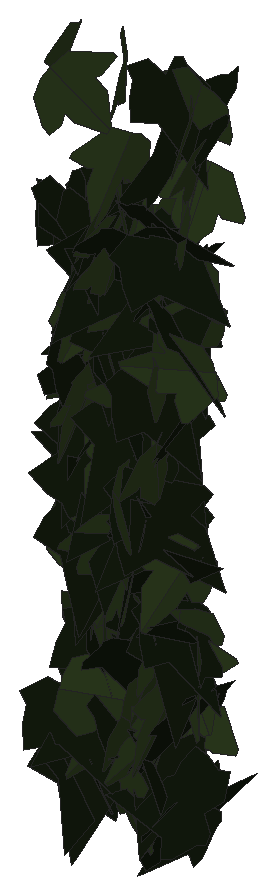
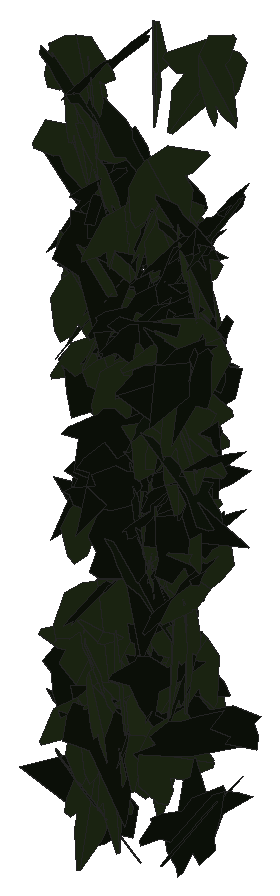
# SketchUp Ruby script. Lengths in inches.
U = 1.inch
M = Sketchup.active_model
def pt(a) = Geom::Point3d.new(a.map { |v| v * U })
def face(e, loops, mat)
  f = e.add_face(loops[0].map { |a| pt(a) })
  loops[1..].each { |l| e.add_face(l.map { |a| pt(a) }).erase! }
  f.material = f.back_material = mat if mat
  f
end
# faces: each face lists its corners as indices into pts; further lists are holes
def faces(e, pts, list, mat = nil) = list.each { |f| face(e, (f[0].is_a?(Array) ? f : [f]).map { |l| l.map { |i| pts[i] } }, mat) }
# xy, xz, yz: faces in a plane at the given z, y or x. An outline is a flat list of corners, or four numbers for a rectangle; further outlines are holes
def ring(l) = l.size == 4 ? [[l[0], l[1]], [l[2], l[1]], [l[2], l[3]], [l[0], l[3]]] : l.each_slice(2).to_a
def flat(e, list, mat, &to3) = list.each { |f| face(e, (f[0].is_a?(Array) ? f : [f]).map { |l| ring(l).map { |u, v| to3.(u, v) } }, mat) }
def xy(e, z, list, mat = nil) = flat(e, list, mat) { |x, y| [x, y, z] }
def xz(e, y, list, mat = nil) = flat(e, list, mat) { |x, z| [x, y, z] }
def yz(e, x, list, mat = nil) = flat(e, list, mat) { |y, z| [x, y, z] }
def lines(e, pts, list) = list.each { |a, b| e.add_line(pt(pts[a]), pt(pts[b])) }
# prism: a flat outline (further loops are holes) pulled along v
def prism(e, loops, v, mat = nil)
  f = face(e, loops, mat); d = Geom::Vector3d.new(v.map { |x| x * U })
  f.pushpull(f.normal.samedirection?(d) ? d.length : -d.length)
end
def box(e, o, s, mat = nil) = prism(e, [[o, [o[0] + s[0], o[1], o[2]], [o[0] + s[0], o[1] + s[1], o[2]], [o[0], o[1] + s[1], o[2]]]], [0, 0, s[2]], mat)
def at(x, y, z, deg = 0) = Geom::Transformation.translation(pt([x, y, z])) * Geom::Transformation.rotation(ORIGIN, Z_AXIS, deg.degrees)
def axes(o, x, y, z) = Geom::Transformation.new([*x, 0, *y, 0, *z, 0, *pt(o).to_a, 1])
def part(name) = M.definitions.add(name)
# library, detail: a bought-in or finely detailed component or shape, given as its bounding box
def library(name, o, s) = part(name).tap { |d| box(d.entities, o, s) }
def detail(e, o, s) = box(e.add_group.entities, o, s)
def put(e, d, t, mat = nil) = e.add_instance(d, t).tap { |i| i.material = mat if mat }
def group(e, t, mat = nil) = e.add_group.tap { |g| g.transformation = t; g.material = mat if mat }.entities
root = M.entities
M.materials.add("efeu1").color = [18, 25, 13]
M.materials.add("efeu2").color = [43, 57, 29]
c1 = part("ivyleaf_10")
p = [[0,0.5,-0.03],[-0.0625,2.02,-0.43],[-0.19,2.01,-0.46],[-0.54,1.05,-0.29],[-0.52,0.625,-0.18],[-0.83,0.76,-0.28],
  [-1.16,0.64,-0.33],[-1.15,0.33,-0.24],[-0.77,-0.39,0.02],[-0.3,-0.51,0.16],[0.04,-0.48,0.23],[-0.02,2.01,-0.4375],
  [-0.06,2.01,-0.43],[0.04,-0.49,0.23],[0.67,-0.49,0.14],[1.38,0.36,-0.2],[1.375,0.51,-0.24],[0.81,0.65,-0.19],
  [0.62,0.59,-0.15],[0.6,1.09,-0.28],[0.5,1.23,-0.31]]
faces(c1.entities,p,[[0,1,2,3,4,5,6,7,8,9,10],[11,12,0,13,14,15,16,17,18,19,20]],"efeu2")
c2 = part("ivyleaf_9")
p = [[1.54,2.16,1.25],[1.36,2.04,1.19],[-0.21,0.99,0.68],[-0.71,1.11,0.82],[-0.85,0.86,0.67],[-0.8,0.17,0.21],
  [-0.9,-0.01,0.1],[-0.67,-0.16,-0.02],[-0.08,-0.08,-0.05],[-0.03,-0.6,-0.4],[0.65,-0.88,-0.66],[0.83,-0.6,-0.49],
  [1.29,-0.42,-0.43],[1.8125,-0.07,-0.26],[1.21,0.44,0.15]]
faces(c2.entities,p,[[0,1,2,3,4,5,6,7,8,9,10,11,12,13,14]],"efeu1")
put(root,c1,axes([29.95,223.1,233.6],[0.17956,-0.41582,0.21179],[0.08166,-0.19542,-0.45293],[0.45945,0.19724,-0.00227]))
put(root,c1,axes([30.06,223.42,228.89],[-0.05304,-0.49708,-0.00977],[0.00051,0.00977,-0.4999],[0.49718,-0.05304,-0.00053]))
put(root,c2,axes([30.42,223.41,227.52],[-0.25058,-0.02517,-0.43194],[-0.40049,-0.17544,0.24256],[-0.16377,0.46753,0.06776]))
put(root,c2,axes([29.98,223.16,227.73],[-0.20354,0.45626,0.01993],[0.00548,-0.01938,0.49959],[0.45666,0.20359,0.00289]))
put(root,c2,axes([29.84,223.58,222.96],[-0.12458,-0.08811,0.47615],[0.1884,-0.46173,-0.03615],[0.44608,0.17041,0.14825]))
put(root,c1,axes([30.21,223.66,228.65],[0.24013,0.26619,-0.34854],[-0.27831,-0.21461,-0.35565],[-0.33894,0.36481,0.0451]))
put(root,c1,axes([30.18,223.21,225.68],[0.24758,-0.24479,-0.35886],[-0.11884,0.35913,-0.32696],[0.41783,0.24719,0.11965]))
put(root,c2,axes([30.04,223.47,226.84],[0.11035,0.19641,0.44637],[-0.21265,-0.39247,0.22527],[0.43886,-0.23956,-0.00308]))
put(root,c2,axes([29.94,223.46,223.11],[-0.02301,-0.43317,0.24866],[0.0184,-0.24949,-0.43292],[0.49913,-0.01077,0.02743]))
put(root,c2,axes([30.07,223.29,229.57],[0.41769,-0.02027,-0.27409],[-0.27364,0.01578,-0.41818],[0.02561,0.49934,0.00209]))
put(root,c1,axes([30.05,223.09,226.37],[0.15967,0.31429,-0.35458],[0.11166,0.33867,0.35048],[0.46047,-0.19111,0.03796]))
put(root,c2,axes([30.04,223.49,223.34],[-0.1616,-0.47288,-0.01649],[0.00518,0.01566,-0.49973],[0.47314,-0.16168,-0.00016]))
put(root,c2,axes([30.15,222.78,229.64],[0.16933,-0.13799,-0.44976],[-0.33041,0.30539,-0.21809],[0.3349,0.37107,0.01224]))
put(root,c1,axes([30.2,223.375,228.5625],[-0.13945,-0.47432,-0.07468],[0.01827,0.07247,-0.49438],[0.47981,-0.14061,-0.00288]))
put(root,c2,axes([30.09,223.54,227.98],[-0.16657,-0.45935,0.10608],[-0.01049,-0.10887,-0.48789],[0.47132,-0.16476,0.02663]))
put(root,c1,axes([30.07,223.27,225.47],[-0.45536,0.10859,-0.17565],[0.17071,-0.04137,-0.46813],[-0.1162,-0.48631,0.00061]))
put(root,c2,axes([29.99,223,231.45],[0.18271,-0.43394,-0.16826],[-0.06692,0.15438,-0.47084],[0.46058,0.19458,-0.00166]))
put(root,c2,axes([30.23,223.02,229.76],[0.1083,0.43687,0.21776],[0.06355,0.20854,-0.44997],[-0.48397,0.12515,-0.01036]))
put(root,c1,axes([30.15,223.2,228.72],[0.14303,-0.39362,0.27314],[0.1033,-0.25301,-0.4187],[0.46784,0.17621,0.00894]))
put(root,c2,axes([30.05,222.95,228.74],[0.05195,0.05503,0.49424],[0.37365,0.3236,-0.0753],[-0.32816,0.37717,-0.0075]))
put(root,c2,axes([29.96,223.0625,231.23],[0.19379,-0.45048,0.09754],[0.04777,-0.08561,-0.49029],[0.45844,0.19935,0.00986]))
put(root,c1,axes([30.3,223.14,231.11],[0.19653,-0.45034,-0.09258],[-0.02909,0.0883,-0.49128],[0.45883,0.19849,0.00851]))
put(root,c1,axes([30.3,223.31,225.67],[0.29723,-0.29937,-0.26838],[-0.04725,0.30544,-0.39303],[0.39928,0.259,0.15328]))
put(root,c2,axes([30.39,223.53,224.19],[-0.29982,-0.30755,0.25597],[-0.14965,-0.21046,-0.42815],[0.3711,-0.33335,0.03415]))
put(root,c1,axes([30.24,223.28,227.25],[-0.45105,0.18806,-0.10578],[0.08147,-0.07854,-0.48703],[-0.1998,-0.45658,0.04021]))
put(root,c1,axes([30,223.23,229.77],[-0.15192,-0.1475,-0.45295],[0.42452,0.17377,-0.19897],[0.21611,-0.44503,0.07243]))
put(root,c2,axes([30.17,223.48,226.33],[-0.04641,-0.46635,0.17424],[-0.02338,-0.17276,-0.46862],[0.49729,-0.05164,-0.00577]))
put(root,c2,axes([30.31,223.36,230.48],[-0.02249,-0.01895,0.49913],[-0.20787,-0.45396,-0.0266],[0.45418,-0.20871,0.01254]))
put(root,c2,axes([30.53,223.02,227.57],[-0.40176,-0.2806,0.09924],[0.08847,0.04659,0.4899],[-0.28418,0.41121,0.01222]))
put(root,c2,axes([30.15,223.46,224.95],[-0.04762,-0.10315,0.48692],[0.07221,-0.4854,-0.09577],[0.49246,0.0612,0.06113]))
put(root,c2,axes([30.22,223.67,229.62],[-0.10238,-0.48585,-0.05891],[0.02217,0.05552,-0.49641],[0.4889,-0.10425,0.01017]))
put(root,c2,axes([30.13,222.9,224.45],[-0.09388,-0.32662,-0.36675],[0.22877,0.30131,-0.32691],[0.43457,-0.22919,0.09287]))
put(root,c2,axes([30.16,223.23,231.24],[0.15216,-0.45216,-0.14967],[0.00274,0.15795,-0.47439],[0.47628,0.14354,0.05055]))
put(root,c1,axes([30.27,222.57,233.34],[0.16339,0.34872,0.3189],[0.04843,0.3233,-0.37833],[-0.47006,0.15452,0.07187]))
put(root,c2,axes([30.6875,222.71,231.1],[-0.21818,0.42155,0.15715],[-0.07105,0.14018,-0.47466],[-0.44424,-0.22945,-0.00127]))
put(root,c2,axes([30.3125,223.07,226.82],[-0.0377,-0.49329,0.07243],[0.00848,-0.07326,-0.49453],[0.4985,-0.03605,0.01389]))
put(root,c1,axes([30.49,223.46,223.96],[-0.02877,-0.19975,0.45746],[0.03516,-0.4579,-0.19773],[0.49793,0.02079,0.0404]))
put(root,c2,axes([30.55,223.36,231.59],[-0.46823,-0.06584,-0.16257],[0.16077,0.02417,-0.47283],[0.07012,-0.49506,-0.00146]))
put(root,c2,axes([30.32,223.47,225.23],[-0.19383,-0.37252,-0.2714],[0.16139,0.22093,-0.4185],[0.43172,-0.24984,0.03459]))
put(root,c1,axes([30.51,223.45,232.07],[-0.14694,-0.4123,0.2417],[0.05078,-0.2649,-0.42101],[0.47521,-0.09918,0.11972]))
put(root,c1,axes([30.58,222.96,230.3125],[0.18998,0.36885,-0.27903],[-0.1809,-0.21836,-0.41182],[-0.42566,0.25742,0.05049]))
put(root,c2,axes([30.82,223.64,229.8],[-0.43342,-0.08519,0.23429],[-0.21463,-0.1115,-0.43761],[0.12681,-0.47991,0.06009]))
put(root,c2,axes([30.56,223.44,227.36],[-0.18521,-0.387,0.25677],[-0.05096,-0.25783,-0.42535],[0.46163,-0.18373,0.05606]))
put(root,c1,axes([30.86,222.97,227.93],[-0.40775,0.09412,0.27364],[-0.28299,-0.22845,-0.34311],[0.06044,-0.43469,0.23957]))
put(root,c1,axes([30.67,223.11,231.15],[0.0333,-0.48236,0.12736],[0.01141,-0.12687,-0.4835],[0.49876,0.03511,0.00256]))
put(root,c2,axes([30.65,223.17,230.62],[-0.22704,-0.37585,0.23915],[-0.06106,-0.23962,-0.43457],[0.44127,-0.22654,0.06291]))
put(root,c1,axes([30.73,223.13,226.31],[0.37861,-0.29117,-0.14789],[-0.11837,0.08868,-0.47762],[0.30437,0.39668,-0.00178]))
put(root,c2,axes([30.52,223.62,230.07],[-0.03628,-0.49232,-0.07942],[0.01755,0.07832,-0.49352],[0.49837,-0.0386,0.01159]))
put(root,c1,axes([30.36,222.8,224.62],[-0.06376,-0.11455,-0.48251],[0.44344,0.20462,-0.10718],[0.22202,-0.4416,0.0755]))
put(root,c1,axes([30.73,222.97,229.56],[-0.2773,0.37834,0.17309],[-0.11412,0.13087,-0.46888],[-0.4001,-0.29955,0.01377]))
put(root,c1,axes([30.75,222.9,227.01],[-0.10633,-0.47185,0.1267],[-0.01697,-0.12602,-0.48356],[0.48827,-0.10714,0.01078]))
put(root,c2,axes([30.63,223.83,230.36],[-0.165,-0.46911,0.05207],[0.00547,-0.05705,-0.4967],[0.47196,-0.16334,0.02396]))
put(root,c2,axes([30.39,223.41,227.34],[0.11293,-0.16673,0.45765],[0.23644,-0.39197,-0.20114],[0.42584,0.26185,-0.00969]))
put(root,c1,axes([30.69,223.68,224.29],[-0.14074,0.21943,-0.42666],[-0.0073,-0.44557,-0.22675],[-0.47973,-0.0576,0.12862]))
put(root,c2,axes([30.47,223.46,228.86],[0.17686,-0.40739,0.22969],[0.07712,-0.21679,-0.44391],[0.46127,0.19244,-0.01384]))
put(root,c1,axes([30.71,223.27,231.39],[-0.22865,0.44121,-0.0552],[0.03582,-0.04359,-0.49681],[-0.44321,-0.23115,-0.01168]))
put(root,c1,axes([30.71,223.03,230.05],[-0.03776,-0.4354,-0.24291],[0.1502,0.22235,-0.4219],[0.47541,-0.10483,0.114]))
put(root,c1,axes([30.81,222.89,230.91],[0.04232,-0.49502,0.05622],[0.01311,-0.0553,-0.49676],[0.49803,0.04352,0.0083]))
put(root,c1,axes([30.85,223.02,233.64],[0.21866,-0.37198,-0.25261],[-0.05681,0.2558,-0.42584],[0.44605,0.21493,0.0696]))
put(root,c2,axes([30.73,222.98,227.38],[-0.35534,-0.21393,-0.27923],[0.22931,0.1601,-0.41447],[0.26674,-0.42261,-0.01567]))
put(root,c1,axes([31.01,222.86,226.42],[-0.04389,0.08644,-0.49051],[-0.17696,0.45758,0.09647],[0.46557,0.18207,-0.00957]))
put(root,c2,axes([30.91,222.97,226.59],[0.36973,0.15023,-0.30122],[-0.28633,-0.09486,-0.39877],[-0.17696,0.46737,0.01589]))
put(root,c2,axes([30.65,223.05,224.31],[0.34491,-0.34306,-0.11553],[-0.06619,0.09712,-0.48599],[0.35589,0.35054,0.02158]))
put(root,c1,axes([30.59,223.41,227.68],[0.13178,-0.17725,0.44857],[0.39436,-0.22813,-0.206],[0.27769,0.4081,0.07967]))
put(root,c2,axes([30.71,223.16,229.88],[0.03438,-0.49878,0.00593],[0.00046,-0.00591,-0.49996],[0.49882,0.03438,0.00006]))
put(root,c1,axes([31.05,223.1875,228.9],[-0.39227,-0.29276,0.10206],[-0.08439,-0.05755,-0.48946],[0.29833,-0.40122,-0.00427]))
put(root,c2,axes([31.26,223.01,226.17],[-0.33083,0.3576,0.11258],[-0.07676,0.08236,-0.48716],[-0.36696,-0.33962,0.00041]))
put(root,c2,axes([31.03,223.23,228.41],[-0.34555,-0.35773,0.05122],[-0.03342,-0.03893,-0.49736],[0.35983,-0.34715,0.00299]))
put(root,c2,axes([31.23,222.71,231.4],[0.16206,0.4123,-0.23183],[-0.14864,-0.18826,-0.43871],[-0.44905,0.21111,0.06156]))
put(root,c1,axes([31.08,223.37,231.23],[0.06713,0.48699,-0.09127],[-0.06543,-0.08259,-0.48877],[-0.49113,0.07757,0.05264]))
put(root,c1,axes([31.22,222.55,227.73],[-0.19417,0.32646,0.32515],[-0.19911,0.25875,-0.37869],[-0.41551,-0.27654,0.02952]))
put(root,c1,axes([31.35,223.33,223.41],[-0.34151,0.16474,0.32593],[-0.30401,0.11901,-0.3787],[-0.20235,-0.45683,0.01888]))
put(root,c1,axes([31.38,222.86,225.58],[0.0748,-0.10529,-0.48303],[-0.31188,0.369,-0.12873],[0.38358,0.32055,-0.01047]))
put(root,c1,axes([30.91,222.91,223.5],[-0.29692,0.1877,-0.35582],[0.28092,-0.21982,-0.35038],[-0.28796,-0.40798,0.02508]))
put(root,c1,axes([31.22,222.59,224.625],[0.0124,-0.31981,-0.38415],[-0.01176,0.38397,-0.32004],[0.49971,0.01698,0.002]))
put(root,c1,axes([31.26,223.15,225.03],[0.1259,-0.42829,-0.2252],[-0.06222,0.21644,-0.44641],[0.47987,0.14044,0.0012]))
put(root,c2,axes([31.13,223.0625,227.16],[-0.24125,0.07491,-0.43149],[0.39802,-0.168,-0.2517],[-0.18269,-0.46494,0.02143]))
put(root,c2,axes([31.34,222.63,225.72],[0.14031,0.46061,-0.13474],[-0.05233,-0.12486,-0.48132],[-0.47705,0.14917,0.01317]))
put(root,c2,axes([31.41,223.28,224.2],[-0.09144,0.49079,-0.02758],[0.00601,-0.02693,-0.49924],[-0.49153,-0.09163,-0.00097]))
put(root,c1,axes([31.35,222.87,230.78],[-0.04289,0.42897,-0.25328],[-0.05788,0.2482,0.43017],[0.49478,0.06622,0.02836]))
put(root,c2,axes([31.5,223.19,232.47],[-0.39828,0.29636,-0.05954],[0.03721,-0.04968,-0.49613],[-0.29998,-0.39963,0.01752]))
put(root,c2,axes([31.05,223.4,228.42],[-0.01416,-0.37865,-0.32623],[0.11585,0.31498,-0.37063],[0.48619,-0.08608,0.07881]))
put(root,c1,axes([31.41,223.23,224.26],[-0.05255,-0.28868,0.40485],[-0.09679,-0.39337,-0.29307],[0.48772,-0.10917,-0.01454]))
put(root,c2,axes([31.46,223.375,227.35],[-0.38974,-0.2895,0.11954],[-0.08808,-0.08183,-0.48533],[0.30057,-0.39937,0.01278]))
put(root,c1,axes([31.37,223.54,224.57],[0.1721,-0.46873,-0.02596],[-0.00691,0.02512,-0.49932],[0.4694,0.17223,0.00217]))
put(root,c2,axes([31.5,223.22,230.68],[-0.02147,0.49525,0.06534],[0.00853,0.06575,-0.49558],[-0.49947,-0.02016,-0.01127]))
put(root,c2,axes([31.09,223.28,223.91],[0.09363,-0.34509,0.3495],[0.12407,-0.32764,-0.35674],[0.47523,0.15352,0.02428]))
put(root,c1,axes([31.48,223.375,225.73],[-0.3903,-0.30246,0.07862],[-0.05781,-0.05375,-0.49373],[0.30712,-0.3945,0.00699]))
put(root,c2,axes([31.62,223.38,230.43],[-0.45216,-0.14212,0.15924],[-0.13611,-0.09533,-0.47158],[0.16441,-0.4698,0.04752]))
put(root,c2,axes([31.26,223.01,227.86],[0.06258,-0.33126,-0.36926],[-0.07739,0.36111,-0.33706],[0.48999,0.09934,-0.00608]))
put(root,c1,axes([31.41,223.39,223.97],[0.01018,-0.47143,0.16629],[0.03332,-0.16531,-0.4707],[0.49878,0.02066,0.02805]))
put(root,c2,axes([31.06,223.06,226.53],[0.12197,-0.15582,0.45918],[0.44001,-0.16339,-0.17232],[0.20375,0.44612,0.09727]))
put(root,c1,axes([31.52,223.39,223.14],[-0.06635,-0.4447,-0.21872],[0.02565,0.2173,-0.44958],[0.49491,-0.07087,-0.00602]))
put(root,c1,axes([31.48,223.6,224.02],[-0.04991,-0.33556,0.3673],[0.09537,-0.36875,-0.32393],[0.48828,0.03772,0.10081]))
put(root,c1,axes([31.47,223.34,229.3125],[0.27642,0.39102,-0.14384],[-0.08508,-0.11601,-0.47886],[-0.40786,0.28921,0.0024]))
put(root,c2,axes([31.28,223.37,233.39],[0.14835,-0.46612,-0.10355],[0.02858,0.11691,-0.4853],[0.47663,0.13807,0.06134]))
put(root,c2,axes([31.34,222.88,229.34],[0.14475,-0.38849,-0.27951],[-0.04057,0.281,-0.41157],[0.47687,0.14183,0.04983]))
put(root,c2,axes([31.3,223.66,229.99],[0.15943,-0.46811,0.07384],[0.03145,-0.06728,-0.49445],[0.47285,0.16231,0.00799]))
put(root,c1,axes([31.58,222.75,228.4375],[0.01645,-0.47591,-0.15246],[0.01601,0.15296,-0.47576],[0.49947,0.01077,0.02027]))
put(root,c1,axes([31.56,223.55,224.3125],[0.26459,0.36104,-0.22281],[-0.12152,-0.18709,-0.44747],[-0.40648,0.29094,-0.01126]))
put(root,c2,axes([31.54,223.15,224.09],[-0.39523,-0.24542,-0.18321],[0.15758,0.09351,-0.46521],[0.26261,-0.42547,0.00343]))
put(root,c1,axes([31.67,223.46,230.08],[-0.18024,-0.40767,0.22654],[-0.07298,-0.21523,-0.44537],[0.46064,-0.19361,0.01808]))
put(root,c1,axes([31.53,223.03,224.79],[0.09375,-0.39981,0.28524],[0.08272,-0.27339,-0.41038],[0.48412,0.12414,0.01489]))
put(root,c1,axes([31.57,222.85,229.64],[0.10342,-0.22734,-0.43315],[0.03396,0.445,-0.22544],[0.48801,0.01721,0.10748]))
put(root,c1,axes([31.78,223.42,233.28],[-0.45998,0.05734,0.18744],[-0.19444,-0.07315,-0.4548],[-0.02474,-0.49129,0.08959]))
put(root,c1,axes([31.63,223.17,231.625],[0.37602,-0.31737,-0.08882],[-0.05421,0.07335,-0.49161],[0.32507,0.37934,0.02075]))
put(root,c1,axes([31.7,223.24,232.99],[0.20574,-0.38373,-0.24582],[-0.09328,0.22854,-0.43482],[0.44606,0.22478,0.02245]))
put(root,c2,axes([31.42,222.94,227.53],[0.05664,-0.28042,-0.41007],[0.02608,0.41384,-0.27939],[0.4961,0.01026,0.06151]))
put(root,c2,axes([31.43,223.22,225.92],[0.20876,-0.4057,-0.20452],[-0.05298,0.2018,-0.45439],[0.45124,0.21139,0.04126]))
put(root,c1,axes([31.62,223.5625,230.59],[0.47069,-0.16757,-0.01934],[-0.0178,0.00769,-0.49962],[0.16774,0.47102,0.00128]))
put(root,c1,axes([31.46,223.4,225.17],[0.38014,0.25344,0.20313],[0.16187,0.12328,-0.45673],[-0.28159,0.413,0.01168]))
put(root,c2,axes([31.82,223.14,228.89],[-0.25541,0.38166,-0.19774],[0.11364,-0.16187,-0.45922],[-0.41455,-0.27952,-0.00406]))
put(root,c1,axes([31.75,223.16,226.78],[-0.22255,-0.32112,0.31202],[-0.02266,-0.33991,-0.36599],[0.44717,-0.17704,0.13674]))
put(root,c2,axes([31.27,223.12,231.33],[0.20262,-0.24376,0.38669],[0.37169,-0.15835,-0.29458],[0.26608,0.40682,0.11704]))
put(root,c2,axes([31.93,223.375,223.24],[-0.45687,0.19949,-0.03842],[0.03608,-0.01336,-0.49852],[-0.19992,-0.45829,-0.00219]))
put(root,c2,axes([31.56,222.88,222.88],[0.03087,0.43552,-0.24365],[-0.03744,0.24545,0.434],[0.49764,-0.00855,0.04776]))
put(root,c2,axes([31.9,223.17,224.79],[-0.19564,0.35288,-0.2953],[0.06392,-0.29693,-0.39718],[-0.45568,-0.19316,0.07107]))
put(root,c2,axes([31.5,222.82,231.38],[0.16037,-0.31358,-0.35489],[0.01049,0.37695,-0.32833],[0.47347,0.09786,0.12749]))
put(root,c2,axes([31.59,223.26,225.64],[-0.00515,-0.49843,0.03931],[-0.00234,-0.03929,-0.49845],[0.49997,-0.00531,-0.00193]))
put(root,c2,axes([32.03,223.48,233.13],[-0.41666,0.27336,-0.04082],[0.0203,-0.04338,-0.4977],[-0.27565,-0.4164,0.02506]))
put(root,c1,axes([32.16,222.8125,229.77],[0.0885,0.02466,-0.49149],[-0.49203,-0.00436,-0.08881],[-0.00867,0.49937,0.02349]))
put(root,c1,axes([31.86,223.31,232.59],[0.12117,-0.47811,-0.08203],[-0.02924,0.0772,-0.49314],[0.48421,0.1243,-0.00925]))
put(root,c1,axes([31.56,223.48,225.125],[0.27351,-0.15283,0.38966],[0.34478,-0.18165,-0.31325],[0.23732,0.44005,0.00602]))
put(root,c1,axes([31.83,223.39,232.12],[0.48552,0.08565,-0.0833],[-0.08168,-0.01648,-0.49301],[-0.0872,0.49233,-0.00201]))
put(root,c2,axes([31.58,222.98,230.32],[0.36648,-0.34011,0.00434],[0.00325,-0.00287,-0.49998],[0.34012,0.36649,0.0001]))
put(root,c2,axes([32.27,222.78,223.57],[-0.32658,0.20348,0.31928],[-0.3148,0.08832,-0.37829],[-0.21035,-0.4481,0.07042]))
